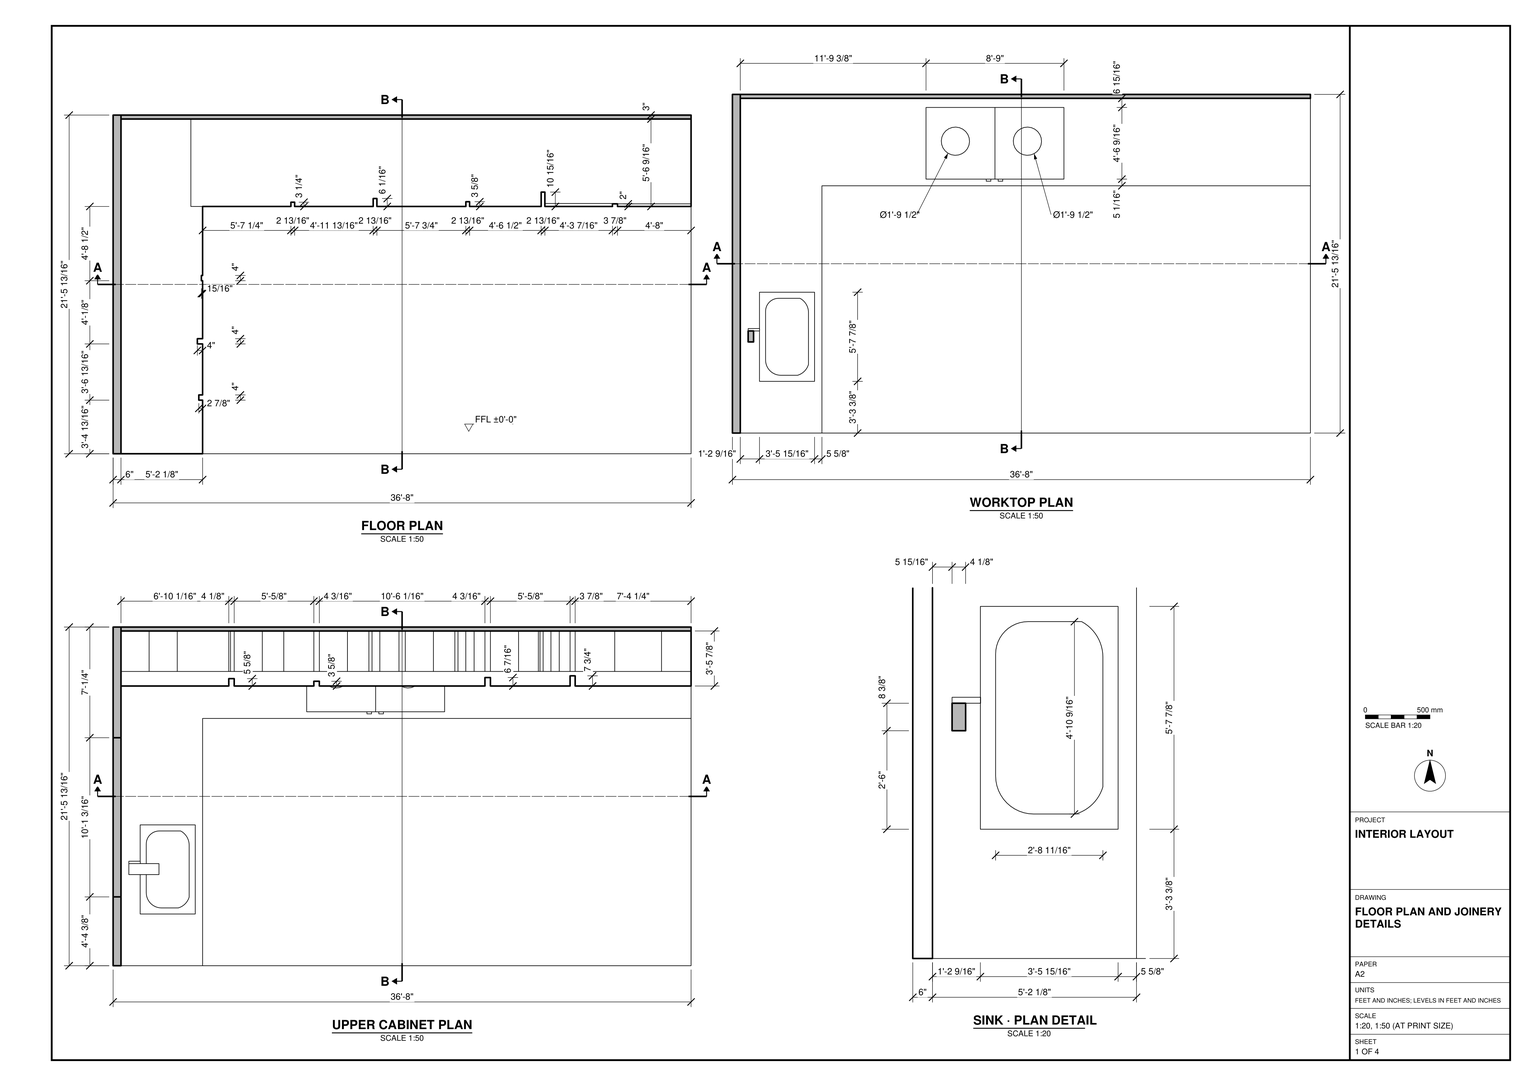
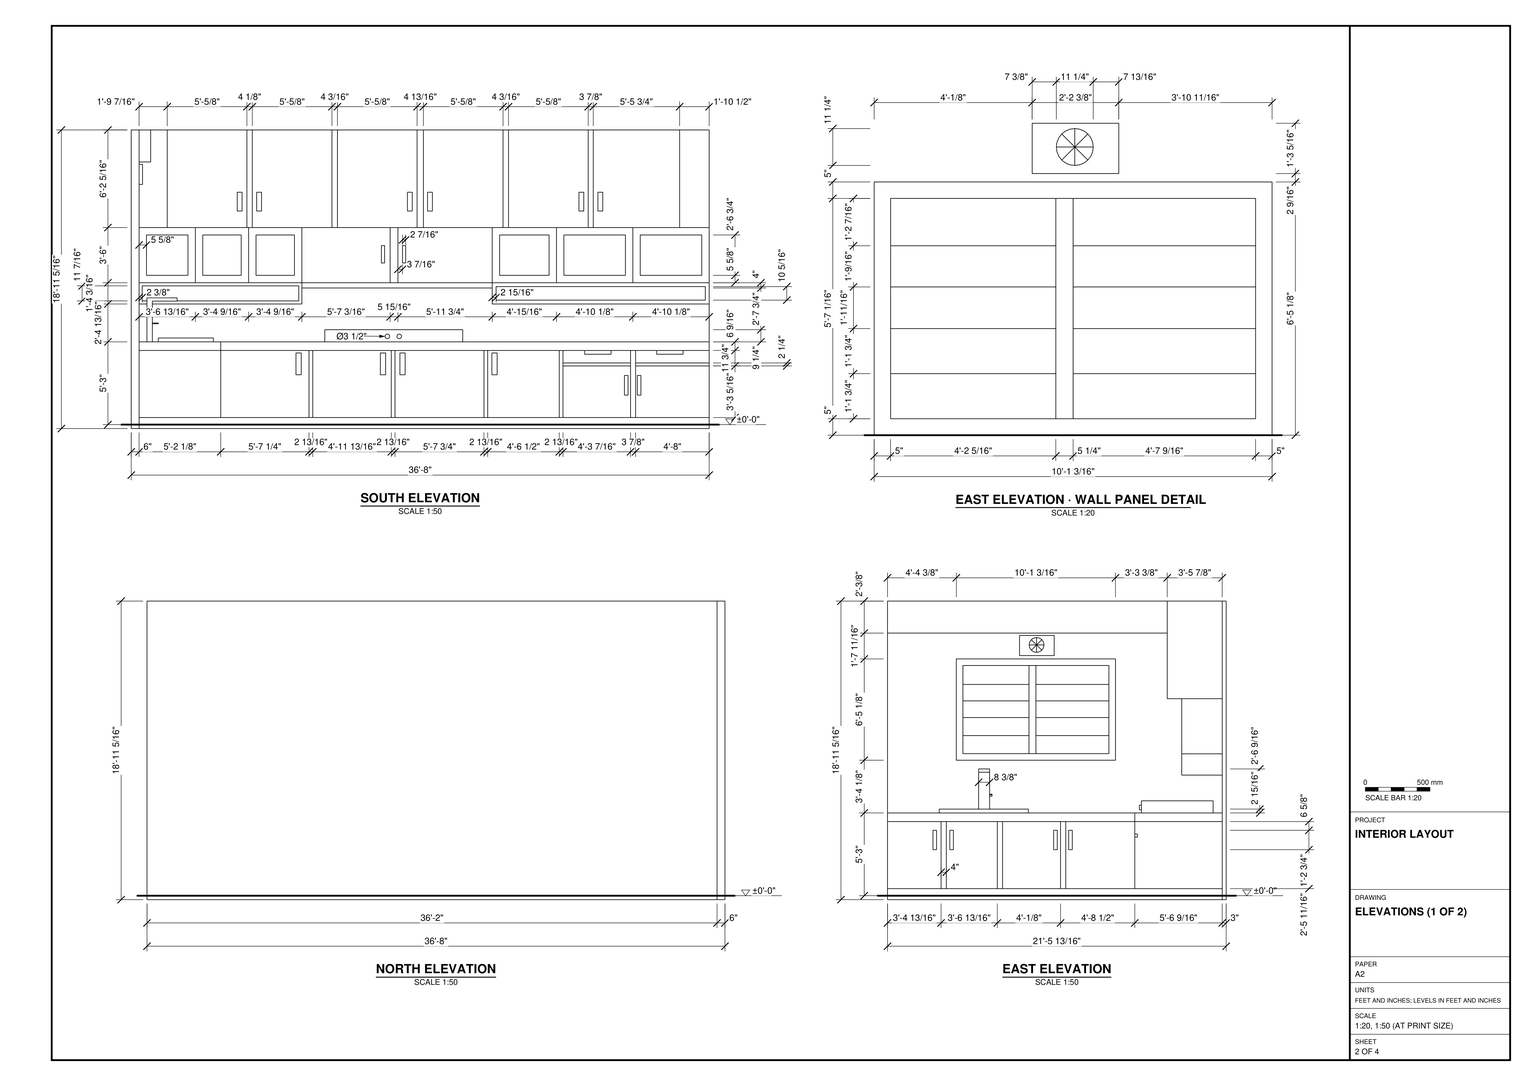
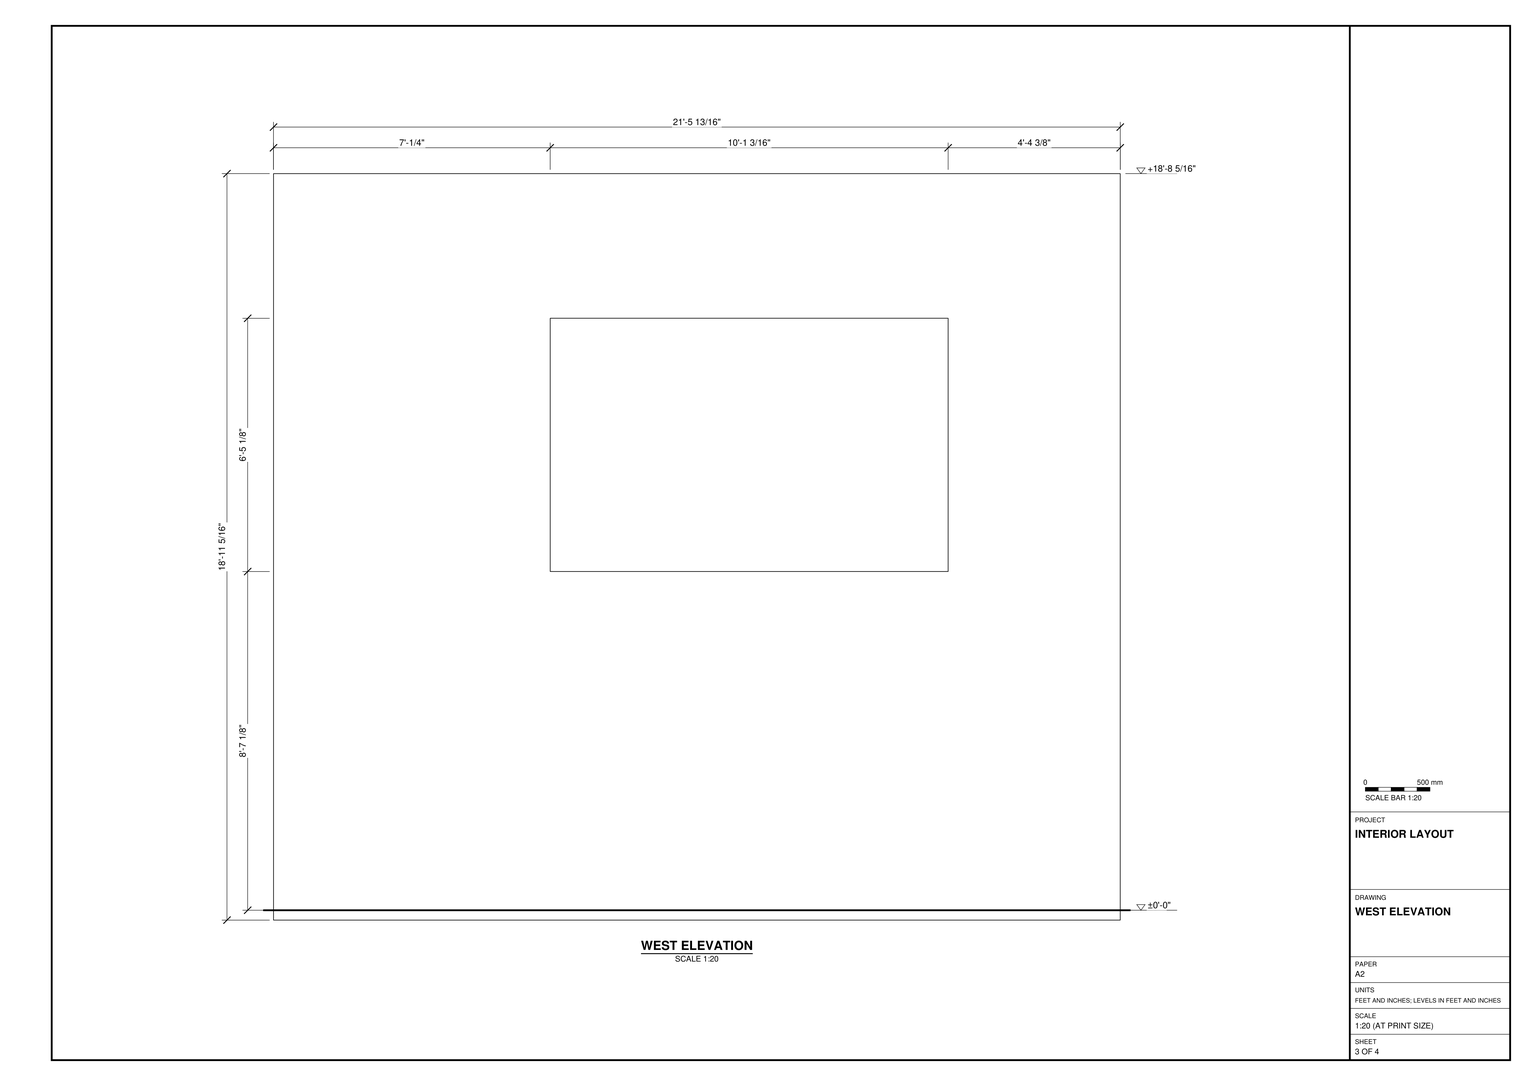
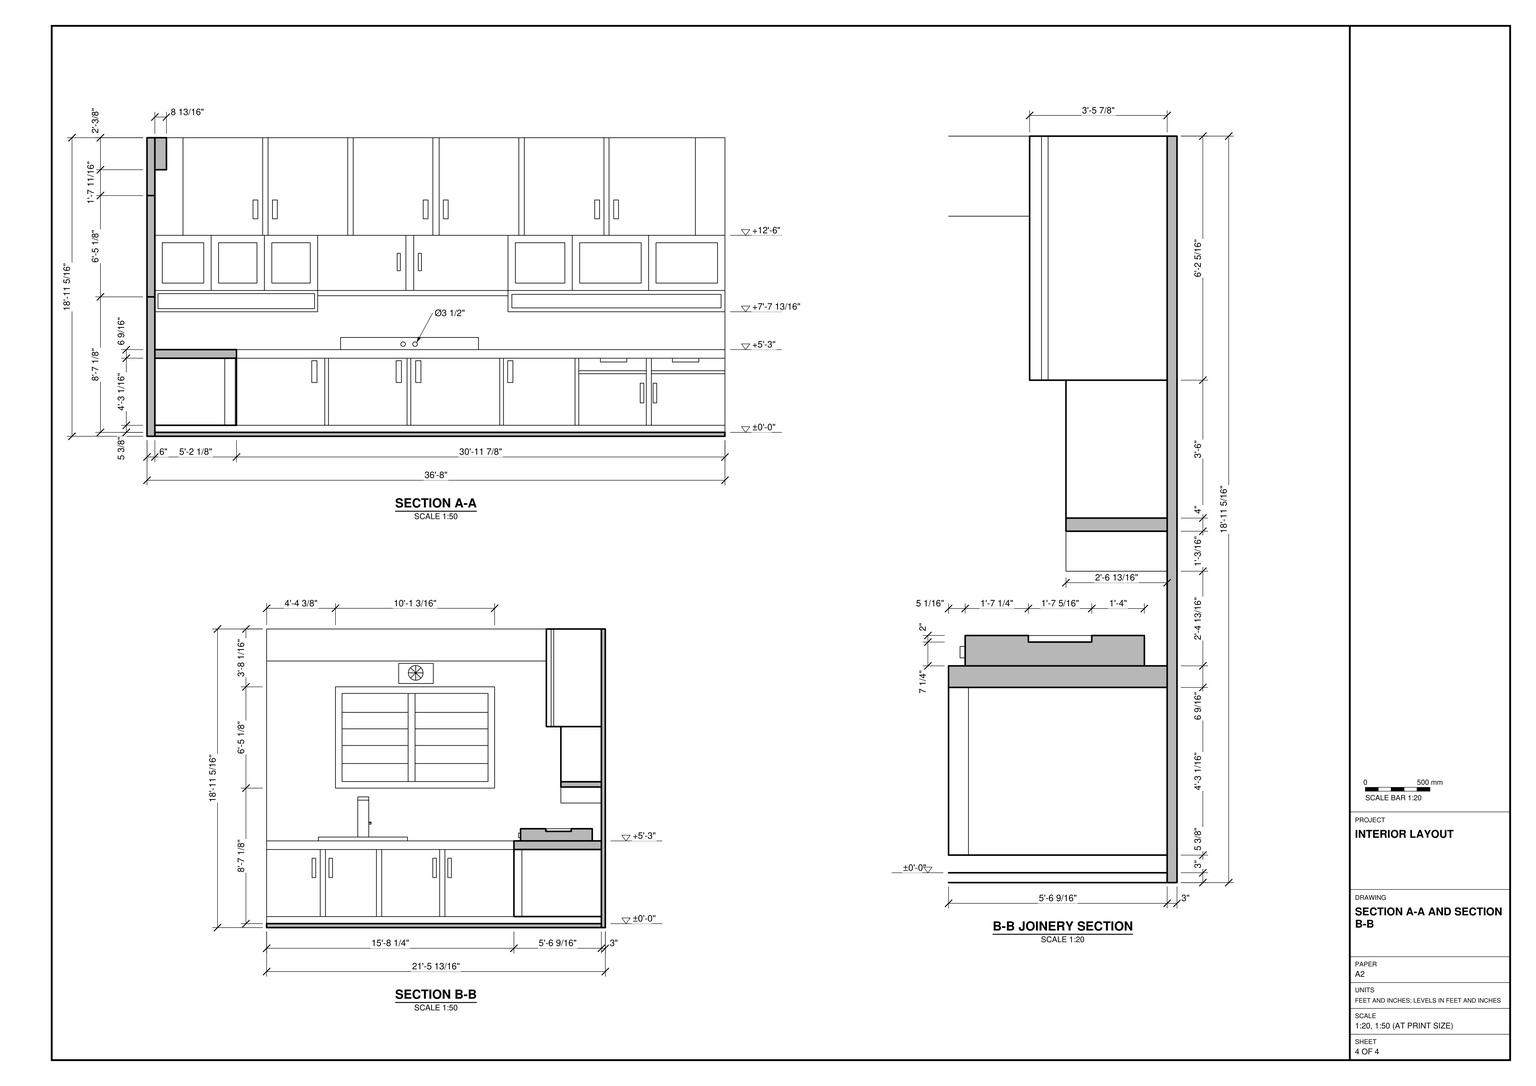
Build the kitchen interior in SketchUp from task_files/diagram_01.pdf. Work in feet and inches. Set the finished floor level to ±0'-0". The overall model extents are 36'-8" along the long cabinet wall, 21'-5 13/16" along the return and 18'-11 5/16" from bottom to top.

Model the rectangular floor slab and the two adjoining walls shown in plan. Make the long back wall 3" thick and the left return wall 6" thick. Follow the floor and worktop plans to form an L-shaped counter with base cabinets beneath both runs. Match the cabinet divisions, plinths, doors, drawer fronts and pulls to the elevations. Place the sink and tap on the return and the cooktop on the long run. Above the sink, model the framed wall panel with its central upright and horizontal divisions, and place the small wall fitting above it.

Use the upper cabinet plan for the depth and spacing of the wall units and the south elevation for their fronts. Distinguish the tall upper doors from the lower tier of framed and plain fronts and the open recesses beneath them. Keep the slab, walls and individual joinery pieces in separate groups or components, and use components for repeated parts. Decor, loose items and appliances may be any suitable library components. Save one SketchUp model as output_files/l_shaped_kitchen_interior_with_fitted_cabinetry.skp.

# SketchUp Ruby script. Lengths in inches.
U = 1.inch
M = Sketchup.active_model
def pt(a) = Geom::Point3d.new(a.map { |v| v * U })
def face(e, loops, mat)
  f = e.add_face(loops[0].map { |a| pt(a) })
  loops[1..].each { |l| e.add_face(l.map { |a| pt(a) }).erase! }
  f.material = f.back_material = mat if mat
  f
end
# faces: each face lists its corners as indices into pts; further lists are holes
def faces(e, pts, list, mat = nil) = list.each { |f| face(e, (f[0].is_a?(Array) ? f : [f]).map { |l| l.map { |i| pts[i] } }, mat) }
# xy, xz, yz: faces in a plane at the given z, y or x. An outline is a flat list of corners, or four numbers for a rectangle; further outlines are holes
def ring(l) = l.size == 4 ? [[l[0], l[1]], [l[2], l[1]], [l[2], l[3]], [l[0], l[3]]] : l.each_slice(2).to_a
def flat(e, list, mat, &to3) = list.each { |f| face(e, (f[0].is_a?(Array) ? f : [f]).map { |l| ring(l).map { |u, v| to3.(u, v) } }, mat) }
def xy(e, z, list, mat = nil) = flat(e, list, mat) { |x, y| [x, y, z] }
def xz(e, y, list, mat = nil) = flat(e, list, mat) { |x, z| [x, y, z] }
def yz(e, x, list, mat = nil) = flat(e, list, mat) { |y, z| [x, y, z] }
def lines(e, pts, list) = list.each { |a, b| e.add_line(pt(pts[a]), pt(pts[b])) }
# prism: a flat outline (further loops are holes) pulled along v
def prism(e, loops, v, mat = nil)
  f = face(e, loops, mat); d = Geom::Vector3d.new(v.map { |x| x * U })
  f.pushpull(f.normal.samedirection?(d) ? d.length : -d.length)
end
def box(e, o, s, mat = nil) = prism(e, [[o, [o[0] + s[0], o[1], o[2]], [o[0] + s[0], o[1] + s[1], o[2]], [o[0], o[1] + s[1], o[2]]]], [0, 0, s[2]], mat)
def at(x, y, z, deg = 0) = Geom::Transformation.translation(pt([x, y, z])) * Geom::Transformation.rotation(ORIGIN, Z_AXIS, deg.degrees)
def axes(o, x, y, z) = Geom::Transformation.new([*x, 0, *y, 0, *z, 0, *pt(o).to_a, 1])
def part(name) = M.definitions.add(name)
# library, detail: a bought-in or finely detailed component or shape, given as its bounding box
def library(name, o, s) = part(name).tap { |d| box(d.entities, o, s) }
def detail(e, o, s) = box(e.add_group.entities, o, s)
def put(e, d, t, mat = nil) = e.add_instance(d, t).tap { |i| i.material = mat if mat }
def group(e, t, mat = nil) = e.add_group.tap { |g| g.transformation = t; g.material = mat if mat }.entities
root = M.entities
M.materials.add("[Color M00]").color = [255, 255, 255]
M.materials.add("[Color M01]").color = [226, 226, 226]
M.materials.add("[Color M03]").color = [170, 170, 170]
M.materials.add("[Formica Graystone]").color = [149, 146, 135]
M.materials.add("[Formica Laminate Dark]").color = [50, 53, 60]
M.materials.add("[Formica Speckled Grey]").color = [94, 105, 111]
M.materials.add("[Quartz Light Brown]").color = [199, 184, 152]
M.materials.add("[Terrazzo Tile Light]").color = [219, 217, 210]
M.materials.add("[Tile Canvas]").color = [199, 192, 173]
M.materials.add("[Tile Ceramic Natural]").color = [189, 180, 134]
M.materials.add("[Tile Limestone Multi]").color = [199, 173, 118]
M.materials.add("[Translucent Glass Gray]").color = [128, 128, 128]
M.materials["[Translucent Glass Gray]"].alpha = 0.5
M.materials.add("[Translucent Glass Safety]").color = [204, 235, 244]
M.materials["[Translucent Glass Safety]"].alpha = 0.5
M.materials.add("[Wood Bamboo]").color = [177, 105, 43]
M.materials.add("[Wood Cherry Original]").color = [152, 86, 42]
M.materials.add("[Wood Floor Light]").color = [204, 176, 127]
xy(root,0,[[0,0,6,257.82],[6,0,439.97,254.82],[6,254.82,439.97,257.82]])
xy(root,3,[[6,0,439.97,254.82]],"[Tile Ceramic Natural]")
xy(root,8.375,[[6,0,6,254.82,59.1875,254.82,59.1875,188.26,68.125,188.26,68.125,135.72,67.1875,135.72,67.1875,131.74,68.125,131.74,68.125,87.6,64.125,87.6,64.125,83.61,68.125,83.61,68.125,44.78,65.25,44.78,65.25,40.8,68.125,40.8,68.125,0],[59.1875,188.26,59.1875,254.82,439.97,254.82,439.97,188.26,383.97,188.26,383.97,190.26,380.12,190.26,380.12,188.26,328.68,188.26,328.68,199.2,325.86,199.2,325.86,188.26,271.37,188.26,271.37,191.88,268.54,191.88,268.54,188.26,200.81,188.26,200.81,194.32,197.98,194.32,197.98,188.26,138.18,188.26,138.18,191.51,135.36,191.51,135.36,188.26]])
xy(root,47.66,[[328.68,188.26,380.12,190.51],[383.97,188.26,439.97,190.26]],"[Formica Laminate Dark]")
xy(root,49.93,[[328.68,188.26,380.12,190.51],[383.97,188.26,439.97,190.26]],"[Formica Laminate Dark]")
xy(root,50.5,[[36.81,44,49.6,44,50.5625,44.33,51.5,44.73,52.4,45.22,53.25,45.77,54.06,46.4,54.81,47.09,55.5,47.84,56.12,48.64,56.68,49.5,57.16,50.4,57.57,51.33,57.89,52.3,57.89,91.75,57.84,92.86,57.7,93.95,57.45,95.03,57.11,96.07,56.68,97.09,56.16,98.0625,55.55,98.98,54.86,99.85,54.1,100.65,53.27,101.37,52.38,102.02,51.4375,102.59,35.11,102.59,33.82,102.51,32.55,102.25,31.32,101.84,30.17,101.27,29.09,100.55,28.12,99.7,27.27,98.72,26.55,97.65,25.98,96.49,25.56,95.26,25.31,94,25.22,92.71,25.22,55.59,25.32,54.08,25.62,52.59,26.11,51.16,26.78,49.8,27.62,48.54,28.62,47.4,29.76,46.4,31.02,45.55,32.38,44.88,33.8125,44.4,35.3,44.1]])
xy(root,59.4375,[[6,0,6,254.82,439.97,254.82,439.97,188.26,383.97,188.26,383.97,190.26,380.12,190.26,380.12,188.26,328.68,188.26,328.68,199.2,325.86,199.2,325.86,188.26,271.37,188.26,271.37,191.88,268.54,191.88,268.54,188.26,200.81,188.26,200.81,194.32,197.98,194.32,197.98,188.26,138.18,188.26,138.18,191.51,135.36,191.51,135.36,188.26,68.125,188.26,68.125,135.72,67.1875,135.72,67.1875,131.74,68.125,131.74,68.125,87.6,64.125,87.6,64.125,83.61,68.125,83.61,68.125,44.78,65.25,44.78,65.25,40.8,68.125,40.8,68.125,0]],"[Color M03]")
xy(root,59.4375,[[65.25,40.8,68.125,44.78],[64.125,83.61,68.125,87.6],[67.1875,131.74,68.125,135.72],[135.36,188.26,138.18,191.51],[197.98,188.26,200.81,194.32],
  [268.54,188.26,271.37,191.88],[325.86,188.26,328.68,199.2],[380.12,188.26,383.97,190.26]],"[Formica Laminate Dark]")
xy(root,66,[[[20.59,39.37,62.53,107.22],[36.81,44,49.6,44,50.5625,44.33,51.5,44.73,52.4,45.22,53.25,45.77,54.06,46.4,54.81,47.09,55.5,47.84,56.12,48.64,56.68,49.5,57.16,50.4,57.57,51.33,57.89,52.3,57.89,91.75,57.84,92.86,57.7,93.95,57.45,95.03,57.11,96.07,56.68,97.09,56.16,98.0625,55.55,98.98,54.86,99.85,54.1,100.65,53.27,101.37,52.38,102.02,51.4375,102.59,35.11,102.59,33.82,102.51,32.55,102.25,31.32,101.84,30.17,101.27,29.09,100.55,28.12,99.7,27.27,98.72,26.55,97.65,25.98,96.49,25.56,95.26,25.31,94,25.22,92.71,25.22,55.59,25.32,54.08,25.62,52.59,26.11,51.16,26.78,49.8,27.62,48.54,28.62,47.4,29.76,46.4,31.02,45.55,32.38,44.88,33.8125,44.4,35.3,44.1]],[11.97,69.36,16.09,77.74],[147.37,193.32,252.37,247.88]])
xy(root,66,[[[6,0,68.125,0,68.125,188.26,439.97,188.26,439.97,254.82,6,254.82],[147.37,193.32,252.37,247.88],[20.59,39.37,62.53,107.22],[11.97,69.36,16.09,77.74]]],"[Formica Laminate Dark]")
xy(root,68.9375,[[[20.59,39.37,62.53,107.22],[36.81,44,35.3,44.1,33.8125,44.4,32.38,44.88,31.02,45.55,29.76,46.4,28.62,47.4,27.62,48.54,26.78,49.8,26.11,51.16,25.62,52.59,25.32,54.08,25.22,55.59,25.22,92.71,25.31,94,25.56,95.26,25.98,96.49,26.55,97.65,27.27,98.72,28.12,99.7,29.09,100.55,30.17,101.27,31.32,101.84,32.55,102.25,33.82,102.51,35.11,102.59,51.4375,102.59,52.38,102.02,53.27,101.37,54.1,100.65,54.86,99.85,55.55,98.98,56.16,98.0625,56.68,97.09,57.11,96.07,57.45,95.03,57.7,93.95,57.84,92.86,57.89,91.75,57.89,52.3,57.57,51.33,57.16,50.4,56.68,49.5,56.12,48.64,55.5,47.84,54.81,47.09,54.06,46.4,53.25,45.77,52.4,45.22,51.5,44.73,50.5625,44.33,49.6,44]]],"[Formica Graystone]")
xy(root,73.25,[[169.4375,211.46,172.23,211.74,174.85,212.74,177.125,214.39,178.9,216.5625,180.04,219.125,180.49,221.89,180.2,224.6875,179.2,227.31,177.56,229.58,175.38,231.35,172.82,232.5,170.05,232.95,167.26,232.66,164.64,231.66,162.36,230.02,160.59,227.84,159.44,225.28,159,222.51,159.28,219.72,160.28,217.09,161.93,214.82,164.11,213.05,166.67,211.9],[224.25,211.46,227.04,211.74,229.66,212.74,231.9375,214.39,233.71,216.5625,234.86,219.125,235.3,221.89,235.01,224.6875,234.01,227.31,232.37,229.58,230.19,231.35,227.63,232.5,224.86,232.95,222.07,232.66,219.45,231.66,217.17,230.02,215.4,227.84,214.26,225.28,213.81,222.51,214.1,219.72,215.1,217.09,216.74,214.82,218.92,213.05,221.48,211.9]],"[Formica Speckled Grey]")
xy(root,75.25,[[[147.37,193.32,199.87,247.88],[169.4375,211.46,166.67,211.9,164.11,213.05,161.93,214.82,160.28,217.09,159.28,219.72,159,222.51,159.44,225.28,160.59,227.84,162.36,230.02,164.64,231.66,167.26,232.66,170.05,232.95,172.82,232.5,175.38,231.35,177.56,229.58,179.2,227.31,180.2,224.6875,180.49,221.89,180.04,219.125,178.9,216.5625,177.125,214.39,174.85,212.74,172.23,211.74]],[[199.87,193.32,252.37,247.88],[224.25,211.46,221.48,211.9,218.92,213.05,216.74,214.82,215.1,217.09,214.1,219.72,213.81,222.51,214.26,225.28,215.4,227.84,217.17,230.02,219.45,231.66,222.07,232.66,224.86,232.95,227.63,232.5,230.19,231.35,232.37,229.58,234.01,227.31,235.01,224.6875,235.3,221.89,234.86,219.125,233.71,216.5625,231.9375,214.39,229.66,212.74,227.04,211.74]]],"[Formica Graystone]")
xy(root,78.75,[[11.97,77.74,16.09,79.55]])
xy(root,79.75,[[16.09,77.74,20.66,79.55]])
xy(root,80.32,[[11.97,77.74,20.66,79.55]],"[Terrazzo Tile Light]")
xy(root,94.8125,[[6,224.01,129.3125,254.82],[129.3125,224.01,129.91,254.82],[274.81,224.01,439.97,254.82]],"[Wood Cherry Original]")
xy(root,96.99,[[16.09,69.36,34.91,77.74]],"[Terrazzo Tile Light]")
xy(root,97.18,[[8.37,224.01,127.55,254.82]],"[Wood Cherry Original]")
xy(root,97.76,[[277.76,224.01,437.03,254.82]],"[Wood Cherry Original]")
xy(root,99.5,[[11.97,69.36,34.91,77.74]],"[Terrazzo Tile Light]")
xy(root,106.15,[[0,52.4,6,173.57]])
xy(root,107,[[129.91,224.01,274.81,254.82]],"[Color M00]")
xy(root,108.05,[[277.76,224.01,323.74,254.82],[323.74,224.01,381.86,254.82],[381.86,224.01,437.03,254.82]],"[Wood Cherry Original]")
xy(root,108.63,[[8.37,224.01,48.84,254.82],[48.84,224.01,89.375,254.82],[89.375,224.01,127.55,254.82]],"[Wood Cherry Original]")
xy(root,111,[[6,224.01,48.84,254.82],[48.84,224.01,89.375,254.82],[89.375,224.01,129.91,254.82],[129.91,224.01,274.81,254.82],[274.81,224.01,323.74,254.82],
  [323.74,224.01,381.86,254.82],[381.86,224.01,439.97,254.82]])
xy(root,116.64,[[11.64,224.01,43.2,254.82],[54.47,224.01,83.74,254.82],[95.01,224.01,124.28,254.82],[280.45,224.01,318.1,254.82],[329.37,224.01,376.22,254.82],
  [387.49,224.01,434.34,254.82]],"[Wood Bamboo]")
xy(root,147.36,[[11.64,224.01,43.2,254.82],[54.47,224.01,83.74,254.82],[95.01,224.01,124.28,254.82],[280.45,224.01,318.1,254.82],[329.37,224.01,376.22,254.82],
  [387.49,224.01,434.34,254.82]],"[Wood Bamboo]")
xy(root,153,[[6,224.01,27.42,254.82],[27.42,224.01,48.84,254.82],[48.84,224.01,88.0625,254.82],[88.0625,224.01,89.375,254.82],[89.375,224.01,92.17,254.82],
  [92.17,224.01,113.59,254.82],[113.59,224.01,129.91,254.82],[129.91,224.01,152.8125,254.82],[152.8125,224.01,156.98,254.82],[156.98,224.01,178.4,254.82],
  [178.4,224.01,194.73,254.82],[194.73,224.01,197.1,254.82],[197.1,224.01,203.05,254.82],[203.05,224.01,217.625,254.82],[217.625,224.01,222.42,254.82],
  [222.42,224.01,243.84,254.82],[243.84,224.01,260.16,254.82],[260.16,224.01,262.54,254.82],[262.54,224.01,268.49,254.82],[268.49,224.01,274.81,254.82],
  [274.81,224.01,283.0625,254.82],[283.0625,224.01,287.23,254.82],[287.23,224.01,308.65,254.82],[308.65,224.01,323.74,254.82],[323.74,224.01,324.98,254.82],
  [324.98,224.01,327.35,254.82],[327.35,224.01,333.3,254.82],[333.3,224.01,339.63,254.82],[339.63,224.01,347.875,254.82],[347.875,224.01,351.74,254.82],
  [351.74,224.01,381.86,254.82],[381.86,224.01,417.48,254.82],[417.48,224.01,439.97,254.82]])
xy(root,153,[[6,212.95,6,224.01,439.97,224.01,439.97,212.95,351.74,212.95,351.74,220.7,347.875,220.7,347.875,212.95,287.23,212.95,287.23,219.38,283.0625,219.38,283.0625,212.95,156.98,212.95,156.98,216.57,152.8125,216.57,152.8125,212.95,92.17,212.95,92.17,218.57,88.0625,218.57,88.0625,212.95]],"[Wood Bamboo]")
xy(root,183.28,[[0,52.4,6,173.57]])
xy(root,185.83,[[6,100.52,8.625,126.9]],"[Color M01]")
xy(root,201.14,[[6,100.52,8.625,126.9]],"[Color M01]")
xy(root,202.9375,[[6,0,14.8125,212.95]])
xy(root,227.3125,[[6,254.82,439.97,257.82]])
xy(root,227.3125,[[6,0,14.8125,212.95]],"[Color M00]")
xy(root,227.3125,[[0,0,6,257.82]],"[Tile Canvas]")
xy(root,227.3125,[[6,212.95,27.42,254.82],[27.42,212.95,88.0625,254.82],[92.17,212.95,152.8125,254.82],[156.98,212.95,217.625,254.82],[217.625,212.95,222.42,254.82],
  [222.42,212.95,283.0625,254.82],[287.23,212.95,347.875,254.82],[351.74,212.95,417.48,254.82],[417.48,212.95,439.97,254.82],[152.8125,216.57,156.98,254.82],
  [88.0625,218.57,92.17,254.82],[283.0625,219.38,287.23,254.82],[347.875,220.7,351.74,254.82]],"[Wood Bamboo]")
xz(root,0,[[6,202.9375,14.8125,227.3125]],"[Color M00]")
xz(root,0,[[6,59.4375,68.125,66]],"[Formica Laminate Dark]")
xz(root,0,[[0,0,6,227.3125],[6,0,439.97,3]],"[Tile Canvas]")
xz(root,0,[[6,8.375,68.125,59.4375]],"[Wood Cherry Original]")
xz(root,39.37,[[20.59,66,62.53,68.9375]],"[Formica Graystone]")
xz(root,40.8,[[65.25,8.375,68.125,59.4375]],"[Formica Laminate Dark]")
xz(root,44,[[36.81,50.5,49.6,66],[36.81,66,49.6,68.9375]],"[Formica Graystone]")
xz(root,44.78,[[65.25,8.375,68.125,59.4375]],"[Formica Laminate Dark]")
xz(root,52.4,[[0,106.15,6,183.28]])
xz(root,69.36,[[11.97,66,16.09,66,16.09,96.99,34.91,96.99,34.91,99.5,11.97,99.5]],"[Terrazzo Tile Light]")
xz(root,77.74,[[11.97,78.75,16.09,80.32]])
xz(root,77.74,[[11.97,66,16.09,78.75],[16.09,79.75,20.66,80.32],[11.97,80.32,11.97,99.5,34.91,99.5,34.91,96.99,16.09,96.99,16.09,80.32]],"[Terrazzo Tile Light]")
xz(root,79.55,[[11.97,78.75,11.97,80.32,20.66,80.32,20.66,79.75,16.09,79.75,16.09,78.75]],"[Terrazzo Tile Light]")
xz(root,83.61,[[64.125,8.375,68.125,59.4375]],"[Formica Laminate Dark]")
xz(root,87.6,[[64.125,8.375,68.125,59.4375]],"[Formica Laminate Dark]")
xz(root,100.52,[[6,185.83,8.625,201.14]],"[Color M01]")
xz(root,102.59,[[35.11,50.5,51.4375,66],[35.11,66,51.4375,68.9375]],"[Formica Graystone]")
xz(root,107.22,[[20.59,66,62.53,68.9375]],"[Formica Graystone]")
xz(root,126.9,[[6,185.83,8.625,201.14]],"[Color M01]")
xz(root,131.74,[[67.1875,8.375,68.125,59.4375]],"[Formica Laminate Dark]")
xz(root,135.72,[[67.1875,8.375,68.125,59.4375]],"[Formica Laminate Dark]")
xz(root,173.57,[[0,106.15,6,183.28]])
xz(root,188.26,[[68.125,59.4375,439.97,66]],"[Formica Laminate Dark]")
xz(root,188.26,[[[68.125,8.375,135.36,59.4375],[125.43,40.93,129.43,57.55]],[[138.18,8.375,197.98,59.4375],[189.68,40.93,193.68,57.55]],[[200.81,8.375,268.54,59.4375],[204.55,40.93,208.55,57.55]],[[271.37,8.375,325.86,59.4375],[274.55,40.93,278.55,57.55]],[[328.68,8.375,380.12,47.66],[375.47,25.42,378.22,40.42]],
  [[383.97,8.375,439.97,47.66],[385.28,25.42,388.03,40.42]],[328.68,49.93,380.12,49.93,380.12,59.4375,365.3,59.4375,365.3,56.5625,345.17,56.5625,345.17,59.4375,328.68,59.4375],[383.97,49.93,439.97,49.93,439.97,59.4375,420.11,59.4375,420.11,56.5625,399.99,56.5625,399.99,59.4375,383.97,59.4375]],"[Wood Cherry Original]")
xz(root,188.26,[[375.47,25.42,378.22,40.42],[385.28,25.42,388.03,40.42],[125.43,40.93,129.43,57.55],[189.68,40.93,193.68,57.55],[204.55,40.93,208.55,57.55],
  [274.55,40.93,278.55,57.55],[345.17,56.5625,365.3,59.4375],[399.99,56.5625,420.11,59.4375]],"[Wood Floor Light]")
xz(root,190.26,[[380.12,8.375,383.97,59.4375],[383.97,47.66,439.97,49.93]],"[Formica Laminate Dark]")
xz(root,190.51,[[328.68,47.66,380.12,49.93]],"[Formica Laminate Dark]")
xz(root,191.51,[[135.36,8.375,138.18,59.4375]],"[Formica Laminate Dark]")
xz(root,191.75,[[194.97,68.43,195.42,68.49,195.84,68.66,196.21,68.94,196.49,69.3,196.66,69.72,196.72,70.18,196.66,70.63,196.49,71.05,196.21,71.42,195.84,71.69,195.42,71.87,194.97,71.93,194.52,71.87,194.09,71.69,193.73,71.42,193.45,71.05,193.28,70.63,193.22,70.18,193.28,69.72,193.45,69.3,193.73,68.94,194.09,68.66,194.52,68.49],[204.03,68.43,204.49,68.49,204.91,68.66,205.27,68.94,205.55,69.3,205.72,69.72,205.78,70.18,205.72,70.63,205.55,71.05,205.27,71.42,204.91,71.69,204.49,71.87,204.03,71.93,203.58,71.87,203.16,71.69,202.79,71.42,202.52,71.05,202.34,70.63,202.28,70.18,202.34,69.72,202.52,69.3,202.79,68.94,203.16,68.66,203.58,68.49]],"[Formica Laminate Dark]")
xz(root,191.88,[[268.54,8.375,271.37,59.4375]],"[Formica Laminate Dark]")
xz(root,193.32,[[194.97,68.43,194.52,68.49,194.09,68.66,193.73,68.94,193.45,69.3,193.28,69.72,193.22,70.18,193.28,70.63,193.45,71.05,193.73,71.42,194.09,71.69,194.52,71.87,194.97,71.93,195.42,71.87,195.84,71.69,196.21,71.42,196.49,71.05,196.66,70.63,196.72,70.18,196.66,69.72,196.49,69.3,196.21,68.94,195.84,68.66,195.42,68.49],[204.03,68.43,203.58,68.49,203.16,68.66,202.79,68.94,202.52,69.3,202.34,69.72,202.28,70.18,202.34,70.63,202.52,71.05,202.79,71.42,203.16,71.69,203.58,71.87,204.03,71.93,204.49,71.87,204.91,71.69,205.27,71.42,205.55,71.05,205.72,70.63,205.78,70.18,205.72,69.72,205.55,69.3,205.27,68.94,204.91,68.66,204.49,68.49]])
xz(root,193.32,[[[147.37,66,252.37,75.25],[194.97,68.43,194.52,68.49,194.09,68.66,193.73,68.94,193.45,69.3,193.28,69.72,193.22,70.18,193.28,70.63,193.45,71.05,193.73,71.42,194.09,71.69,194.52,71.87,194.97,71.93,195.42,71.87,195.84,71.69,196.21,71.42,196.49,71.05,196.66,70.63,196.72,70.18,196.66,69.72,196.49,69.3,196.21,68.94,195.84,68.66,195.42,68.49],[204.03,68.43,203.58,68.49,203.16,68.66,202.79,68.94,202.52,69.3,202.34,69.72,202.28,70.18,202.34,70.63,202.52,71.05,202.79,71.42,203.16,71.69,203.58,71.87,204.03,71.93,204.49,71.87,204.91,71.69,205.27,71.42,205.55,71.05,205.72,70.63,205.78,70.18,205.72,69.72,205.55,69.3,205.27,68.94,204.91,68.66,204.49,68.49]]],"[Formica Graystone]")
xz(root,194.32,[[197.98,8.375,200.81,59.4375]],"[Formica Laminate Dark]")
xz(root,199.2,[[325.86,8.375,328.68,59.4375]],"[Formica Laminate Dark]")
xz(root,212.95,[[6,202.9375,14.8125,227.3125]])
xz(root,212.95,[[217.625,153,222.42,227.3125]],"[Formica Laminate Dark]")
xz(root,212.95,[[6,153,27.42,153,27.42,227.3125,14.8125,227.3125,14.8125,202.9375,6,202.9375],[[27.42,153,88.0625,227.3125],[80.71,165.59,84.4,179.9]],[[92.17,153,152.8125,227.3125],[95.52,165.59,99.21,179.9]],[[156.98,153,217.625,227.3125],[210.27,165.59,213.96,179.9]],[[222.42,153,283.0625,227.3125],[225.58,165.59,229.27,179.9]],
  [[287.23,153,347.875,227.3125],[340.83,165.59,344.52,179.9]],[[351.74,153,417.48,227.3125],[355.27,165.59,358.96,179.9]],[417.48,153,439.97,227.3125]],"[Wood Bamboo]")
xz(root,212.95,[[80.71,165.59,84.4,179.9],[95.52,165.59,99.21,179.9],[210.27,165.59,213.96,179.9],[225.58,165.59,229.27,179.9],[340.83,165.59,344.52,179.9],
  [355.27,165.59,358.96,179.9]],"[Wood Floor Light]")
xz(root,216.57,[[152.8125,153,156.98,227.3125]],"[Formica Laminate Dark]")
xz(root,218.57,[[88.0625,153,92.17,227.3125]],"[Formica Laminate Dark]")
xz(root,219.38,[[283.0625,153,287.23,227.3125]],"[Formica Laminate Dark]")
xz(root,220.7,[[347.875,153,351.74,227.3125]],"[Formica Laminate Dark]")
xz(root,224.01,[[129.91,107,274.81,111]],"[Color M00]")
xz(root,224.01,[[197.1,111,203.05,153]],"[Formica Laminate Dark]")
xz(root,224.01,[[11.64,116.64,43.2,147.36],[54.47,116.64,83.74,147.36],[95.01,116.64,124.28,147.36],[280.45,116.64,318.1,147.36],[329.37,116.64,376.22,147.36],
  [387.49,116.64,434.34,147.36]],"[Translucent Glass Safety]")
xz(root,224.01,[[[6,111,48.84,153],[11.64,116.64,43.2,147.36]],[[48.84,111,89.375,153],[54.47,116.64,83.74,147.36]],[[89.375,111,129.91,153],[95.01,116.64,124.28,147.36]],[[274.81,111,323.74,153],[280.45,116.64,318.1,147.36]],[[323.74,111,381.86,153],[329.37,116.64,376.22,147.36]],
  [[381.86,111,439.97,153],[387.49,116.64,434.34,147.36]]],"[Wood Bamboo]")
xz(root,224.01,[[[6,94.8125,129.91,111],[8.37,97.18,127.55,108.63]],[[274.81,94.8125,439.97,111],[277.76,97.76,437.03,108.05]],[[129.91,111,197.1,153],[190.46,126.04,192.89,139.29]],[[203.05,111,274.81,153],[206.52,126.04,208.96,139.29]]],"[Wood Cherry Original]")
xz(root,224.01,[[190.46,126.04,192.89,139.29],[206.52,126.04,208.96,139.29]],"[Wood Floor Light]")
xz(root,247.88,[[147.37,66,252.37,75.25]])
xz(root,254.82,[[6,0,439.97,3],[6,8.375,59.1875,59.4375],[59.1875,8.375,439.97,59.4375],[6,59.4375,59.1875,66],[59.1875,59.4375,439.97,66],
  [[6,94.8125,129.91,111],[8.37,97.18,127.55,108.63]],[[274.81,94.8125,439.97,111],[277.76,97.76,437.03,108.05]],[129.91,107,197.1,111],[197.1,107,203.05,111],[203.05,107,274.81,111],
  [[6,111,48.84,153],[11.64,116.64,43.2,147.36]],[[48.84,111,89.375,153],[54.47,116.64,83.74,147.36]],[[89.375,111,129.91,153],[95.01,116.64,124.28,147.36]],[129.91,111,197.1,153],[197.1,111,203.05,153],
  [203.05,111,274.81,153],[[274.81,111,323.74,153],[280.45,116.64,318.1,147.36]],[[323.74,111,381.86,153],[329.37,116.64,376.22,147.36]],[[381.86,111,439.97,153],[387.49,116.64,434.34,147.36]],[6,153,27.42,227.3125],
  [27.42,153,88.0625,227.3125],[88.0625,153,92.17,227.3125],[92.17,153,152.8125,227.3125],[152.8125,153,156.98,227.3125],[156.98,153,217.625,227.3125],
  [217.625,153,222.42,227.3125],[222.42,153,283.0625,227.3125],[283.0625,153,287.23,227.3125],[287.23,153,347.875,227.3125],[347.875,153,351.74,227.3125],
  [351.74,153,417.48,227.3125],[417.48,153,439.97,227.3125]])
xz(root,254.82,[[6,3,439.97,8.375],[6,66,439.97,66,439.97,94.8125,274.81,94.8125,274.81,107,129.91,107,129.91,94.8125,6,94.8125]],"[Tile Canvas]")
xz(root,254.82,[[11.64,116.64,43.2,147.36],[54.47,116.64,83.74,147.36],[95.01,116.64,124.28,147.36],[280.45,116.64,318.1,147.36],[329.37,116.64,376.22,147.36],
  [387.49,116.64,434.34,147.36]],"[Wood Bamboo]")
xz(root,254.82,[[8.37,97.18,127.55,108.63],[277.76,97.76,437.03,108.05]],"[Wood Cherry Original]")
xz(root,257.82,[[0,0,6,227.3125],[6,0,439.97,227.3125]],"[Tile Limestone Multi]")
yz(root,0,[[[0,0,257.82,227.3125],[52.4,106.15,173.57,183.28]],[52.4,106.15,173.57,183.28]],"[Tile Limestone Multi]")
yz(root,6,[[0,0,254.82,3],[254.82,0,257.82,227.3125],[0,8.375,254.82,59.4375],[0,59.4375,254.82,66],[224.01,94.8125,254.82,111],
  [224.01,111,254.82,153],[212.95,153,254.82,227.3125],[0,202.9375,212.95,227.3125]])
yz(root,6,[[100.52,185.83,126.9,201.14]],"[Color M01]")
yz(root,6,[[[52.4,106.15,173.57,183.28],[57.42,111.17,168.55,178.26]],[107.72,111.17,112.98,178.26]],"[Quartz Light Brown]")
yz(root,6,[[0,3,254.82,8.375],[[0,66,254.82,66,254.82,94.8125,224.01,94.8125,224.01,153,212.95,153,212.95,202.9375,0,202.9375],[52.4,106.15,173.57,183.28],[100.52,185.83,126.9,201.14]]],"[Tile Canvas]")
yz(root,6,[[57.42,111.17,107.72,124.9],[112.98,111.17,168.55,124.9],[57.42,124.9,107.72,138.625],[112.98,124.9,168.55,138.625],[57.42,138.625,107.72,151.31],
  [112.98,138.625,168.55,151.31],[57.42,151.31,107.72,163.84],[112.98,151.31,168.55,163.84],[57.42,163.84,107.72,178.26],[112.98,163.84,168.55,178.26]],"[Translucent Glass Gray]")
yz(root,8.37,[[224.01,97.18,254.82,108.63]],"[Wood Cherry Original]")
yz(root,8.625,[[[100.52,185.83,126.9,201.14],[113.49,188.29,112.04,188.49,110.68,189.05,109.51,189.94,108.62,191.11,108.06,192.46,107.87,193.92,108.06,195.375,108.62,196.73,109.51,197.9,110.68,198.79,112.04,199.35,113.49,199.54,114.95,199.35,116.3,198.79,117.47,197.9,118.36,196.73,118.92,195.375,119.12,193.92,118.92,192.46,118.36,191.11,117.47,189.94,116.3,189.05,114.95,188.49]],[113.49,188.29,113.49,193.92,109.51,189.94,110.68,189.05,112.04,188.49],[113.49,188.29,114.95,188.49,116.3,189.05,117.47,189.94,113.49,193.92],[109.51,189.94,113.49,193.92,107.87,193.92,108.06,192.46,108.62,191.11],[117.47,189.94,118.36,191.11,118.92,192.46,119.12,193.92,113.49,193.92],
  [107.87,193.92,113.49,193.92,109.51,197.9,108.62,196.73,108.06,195.375],[113.49,193.92,113.49,199.54,112.04,199.35,110.68,198.79,109.51,197.9],[113.49,193.92,117.47,197.9,116.3,198.79,114.95,199.35,113.49,199.54],[113.49,193.92,119.12,193.92,118.92,195.375,118.36,196.73,117.47,197.9]],"[Color M01]")
yz(root,11.64,[[224.01,116.64,254.82,147.36]],"[Wood Bamboo]")
yz(root,11.97,[[69.36,66,77.74,99.5],[77.74,78.75,79.55,80.32]],"[Terrazzo Tile Light]")
yz(root,14.8125,[[0,202.9375,212.95,227.3125]],"[Color M00]")
yz(root,16.09,[[69.36,66,77.74,96.99],[77.74,78.75,79.55,79.75]],"[Terrazzo Tile Light]")
yz(root,20.59,[[39.37,66,107.22,68.9375]],"[Formica Graystone]")
yz(root,20.66,[[77.74,79.75,79.55,80.32]])
yz(root,25.22,[[55.59,50.5,92.71,66],[55.59,66,92.71,68.9375]],"[Formica Graystone]")
yz(root,34.91,[[69.36,96.99,77.74,99.5]],"[Terrazzo Tile Light]")
yz(root,43.2,[[224.01,116.64,254.82,147.36]],"[Wood Bamboo]")
yz(root,48.84,[[224.01,111,254.82,153]])
yz(root,54.47,[[224.01,116.64,254.82,147.36]],"[Wood Bamboo]")
yz(root,57.89,[[52.3,50.5,91.75,66],[52.3,66,91.75,68.9375]],"[Formica Graystone]")
yz(root,62.53,[[39.37,66,107.22,68.9375]],"[Formica Graystone]")
yz(root,64.125,[[83.61,8.375,87.6,59.4375]],"[Formica Laminate Dark]")
yz(root,65.25,[[40.8,8.375,44.78,59.4375]],"[Formica Laminate Dark]")
yz(root,67.1875,[[131.74,8.375,135.72,59.4375]],"[Formica Laminate Dark]")
yz(root,68.125,[[0,59.4375,188.26,66]],"[Formica Laminate Dark]")
yz(root,68.125,[[[0,8.375,40.8,59.4375],[34.61,38.05,37.36,52.8]],[[44.78,8.375,83.61,59.4375],[47.43,38.05,50.18,52.8]],[[87.6,8.375,131.74,59.4375],[126.49,38.05,129.24,52.8]],[[135.72,8.375,188.26,59.4375],[137.93,38.05,140.68,52.8]]],"[Wood Cherry Original]")
yz(root,68.125,[[34.61,38.05,37.36,52.8],[47.43,38.05,50.18,52.8],[126.49,38.05,129.24,52.8],[137.93,38.05,140.68,52.8]],"[Wood Floor Light]")
yz(root,83.74,[[224.01,116.64,254.82,147.36]],"[Wood Bamboo]")
yz(root,88.0625,[[212.95,153,218.57,227.3125]],"[Formica Laminate Dark]")
yz(root,89.375,[[224.01,111,254.82,153]])
yz(root,92.17,[[212.95,153,218.57,227.3125]],"[Formica Laminate Dark]")
yz(root,95.01,[[224.01,116.64,254.82,147.36]],"[Wood Bamboo]")
yz(root,124.28,[[224.01,116.64,254.82,147.36]],"[Wood Bamboo]")
yz(root,127.55,[[224.01,97.18,254.82,108.63]],"[Wood Cherry Original]")
yz(root,129.91,[[224.01,107,254.82,111],[224.01,111,254.82,153]])
yz(root,129.91,[[224.01,94.8125,254.82,107]],"[Wood Cherry Original]")
yz(root,135.36,[[188.26,8.375,191.51,59.4375]],"[Formica Laminate Dark]")
yz(root,138.18,[[188.26,8.375,191.51,59.4375]],"[Formica Laminate Dark]")
yz(root,147.37,[[193.32,66,247.88,75.25]],"[Formica Graystone]")
yz(root,152.8125,[[212.95,153,216.57,227.3125]],"[Formica Laminate Dark]")
yz(root,156.98,[[212.95,153,216.57,227.3125]],"[Formica Laminate Dark]")
yz(root,197.98,[[188.26,8.375,194.32,59.4375]],"[Formica Laminate Dark]")
yz(root,200.81,[[188.26,8.375,194.32,59.4375]],"[Formica Laminate Dark]")
yz(root,252.37,[[193.32,66,247.88,75.25]],"[Formica Graystone]")
yz(root,268.54,[[188.26,8.375,191.88,59.4375]],"[Formica Laminate Dark]")
yz(root,271.37,[[188.26,8.375,191.88,59.4375]],"[Formica Laminate Dark]")
yz(root,274.81,[[224.01,107,254.82,111],[224.01,111,254.82,153]])
yz(root,274.81,[[224.01,94.8125,254.82,107]],"[Wood Cherry Original]")
yz(root,277.76,[[224.01,97.76,254.82,108.05]],"[Wood Cherry Original]")
yz(root,280.45,[[224.01,116.64,254.82,147.36]],"[Wood Bamboo]")
yz(root,283.0625,[[212.95,153,219.38,227.3125]],"[Formica Laminate Dark]")
yz(root,287.23,[[212.95,153,219.38,227.3125]],"[Formica Laminate Dark]")
yz(root,318.1,[[224.01,116.64,254.82,147.36]],"[Wood Bamboo]")
yz(root,323.74,[[224.01,111,254.82,153]])
yz(root,325.86,[[188.26,8.375,199.2,59.4375]],"[Formica Laminate Dark]")
yz(root,328.68,[[188.26,8.375,199.2,47.66],[190.51,47.66,199.2,49.93],[188.26,49.93,199.2,59.4375]],"[Formica Laminate Dark]")
yz(root,329.37,[[224.01,116.64,254.82,147.36]],"[Wood Bamboo]")
yz(root,347.875,[[212.95,153,220.7,227.3125]],"[Formica Laminate Dark]")
yz(root,351.74,[[212.95,153,220.7,227.3125]],"[Formica Laminate Dark]")
yz(root,376.22,[[224.01,116.64,254.82,147.36]],"[Wood Bamboo]")
yz(root,380.12,[[188.26,8.375,190.26,47.66],[190.26,47.66,190.51,49.93],[188.26,49.93,190.26,59.4375]],"[Formica Laminate Dark]")
yz(root,381.86,[[224.01,111,254.82,153]])
yz(root,383.97,[[188.26,8.375,190.26,47.66],[188.26,49.93,190.26,59.4375]],"[Formica Laminate Dark]")
yz(root,387.49,[[224.01,116.64,254.82,147.36]],"[Wood Bamboo]")
yz(root,434.34,[[224.01,116.64,254.82,147.36]],"[Wood Bamboo]")
yz(root,437.03,[[224.01,97.76,254.82,108.05]],"[Wood Cherry Original]")
yz(root,439.97,[[188.26,59.4375,254.82,66]],"[Formica Laminate Dark]")
yz(root,439.97,[[0,0,254.82,3],[254.82,0,257.82,227.3125]],"[Tile Canvas]")
yz(root,439.97,[[224.01,111,254.82,153],[212.95,153,254.82,227.3125]],"[Wood Bamboo]")
yz(root,439.97,[[188.26,8.375,254.82,8.375,254.82,59.4375,188.26,59.4375,188.26,49.93,190.26,49.93,190.26,47.66,188.26,47.66],[224.01,94.8125,254.82,111]],"[Wood Cherry Original]")
p = [[35.3,44.1,66],[36.81,44,66],[36.81,44,50.5],[35.3,44.1,50.5],[49.6,44,66],[50.5625,44.33,66],
  [50.5625,44.33,50.5],[49.6,44,50.5],[33.8125,44.4,66],[33.8125,44.4,50.5],[51.5,44.73,66],[51.5,44.73,50.5],
  [32.38,44.88,66],[32.38,44.88,50.5],[52.4,45.22,66],[52.4,45.22,50.5],[31.02,45.55,66],[31.02,45.55,50.5],
  [53.25,45.77,66],[53.25,45.77,50.5],[29.76,46.4,66],[29.76,46.4,50.5],[54.06,46.4,66],[54.06,46.4,50.5],
  [28.62,47.4,66],[28.62,47.4,50.5],[54.81,47.09,66],[54.81,47.09,50.5],[55.5,47.84,66],[55.5,47.84,50.5],
  [27.62,48.54,66],[27.62,48.54,50.5],[56.12,48.64,66],[56.12,48.64,50.5],[26.78,49.8,66],[26.78,49.8,50.5],
  [56.68,49.5,66],[56.68,49.5,50.5],[57.16,50.4,66],[57.16,50.4,50.5],[26.11,51.16,66],[26.11,51.16,50.5],
  [57.57,51.33,66],[57.57,51.33,50.5],[25.62,52.59,66],[25.62,52.59,50.5],[57.89,52.3,66],[57.89,52.3,50.5],
  [25.32,54.08,66],[25.32,54.08,50.5],[25.22,55.59,66],[25.22,55.59,50.5],[57.89,91.75,66],[57.84,92.86,66],
  [57.84,92.86,50.5],[57.89,91.75,50.5],[25.31,94,66],[25.22,92.71,66],[25.22,92.71,50.5],[25.31,94,50.5],
  [57.7,93.95,66],[57.7,93.95,50.5],[57.45,95.03,66],[57.45,95.03,50.5],[25.56,95.26,66],[25.56,95.26,50.5],
  [57.11,96.07,66],[57.11,96.07,50.5],[25.98,96.49,66],[25.98,96.49,50.5],[56.68,97.09,66],[56.68,97.09,50.5],
  [26.55,97.65,66],[26.55,97.65,50.5],[56.16,98.0625,66],[56.16,98.0625,50.5],[27.27,98.72,66],[27.27,98.72,50.5],
  [55.55,98.98,66],[55.55,98.98,50.5],[28.12,99.7,66],[28.12,99.7,50.5],[54.86,99.85,66],[54.86,99.85,50.5],
  [29.09,100.55,66],[29.09,100.55,50.5],[54.1,100.65,66],[54.1,100.65,50.5],[30.17,101.27,66],[30.17,101.27,50.5],
  [53.27,101.37,66],[53.27,101.37,50.5],[31.32,101.84,66],[31.32,101.84,50.5],[52.38,102.02,66],[52.38,102.02,50.5],
  [32.55,102.25,66],[32.55,102.25,50.5],[51.4375,102.59,66],[51.4375,102.59,50.5],[33.82,102.51,66],[33.82,102.51,50.5],
  [35.11,102.59,66],[35.11,102.59,50.5],[35.3,44.1,68.9375],[36.81,44,68.9375],[49.6,44,68.9375],[50.5625,44.33,68.9375],
  [33.8125,44.4,68.9375],[51.5,44.73,68.9375],[32.38,44.88,68.9375],[52.4,45.22,68.9375],[31.02,45.55,68.9375],[53.25,45.77,68.9375],
  [29.76,46.4,68.9375],[54.06,46.4,68.9375],[28.62,47.4,68.9375],[54.81,47.09,68.9375],[55.5,47.84,68.9375],[27.62,48.54,68.9375],
  [56.12,48.64,68.9375],[26.78,49.8,68.9375],[56.68,49.5,68.9375],[57.16,50.4,68.9375],[26.11,51.16,68.9375],[57.57,51.33,68.9375],
  [25.62,52.59,68.9375],[57.89,52.3,68.9375],[25.32,54.08,68.9375],[25.22,55.59,68.9375],[57.89,91.75,68.9375],[57.84,92.86,68.9375],
  [25.31,94,68.9375],[25.22,92.71,68.9375],[57.7,93.95,68.9375],[57.45,95.03,68.9375],[25.56,95.26,68.9375],[57.11,96.07,68.9375],
  [25.98,96.49,68.9375],[56.68,97.09,68.9375],[26.55,97.65,68.9375],[56.16,98.0625,68.9375],[27.27,98.72,68.9375],[55.55,98.98,68.9375],
  [28.12,99.7,68.9375],[54.86,99.85,68.9375],[29.09,100.55,68.9375],[54.1,100.65,68.9375],[30.17,101.27,68.9375],[53.27,101.37,68.9375],
  [31.32,101.84,68.9375],[52.38,102.02,68.9375],[32.55,102.25,68.9375],[51.4375,102.59,68.9375],[33.82,102.51,68.9375],[35.11,102.59,68.9375],
  [194.52,193.32,68.49],[194.97,193.32,68.43],[194.97,191.75,68.43],[194.52,191.75,68.49],[195.42,193.32,68.49],[195.42,191.75,68.49],
  [203.58,193.32,68.49],[204.03,193.32,68.43],[204.03,191.75,68.43],[203.58,191.75,68.49],[204.49,193.32,68.49],[204.49,191.75,68.49],
  [194.09,193.32,68.66],[194.09,191.75,68.66],[195.84,193.32,68.66],[195.84,191.75,68.66],[203.16,193.32,68.66],[203.16,191.75,68.66],
  [204.91,193.32,68.66],[204.91,191.75,68.66],[193.73,193.32,68.94],[193.73,191.75,68.94],[196.21,193.32,68.94],[196.21,191.75,68.94],
  [202.79,193.32,68.94],[202.79,191.75,68.94],[205.27,193.32,68.94],[205.27,191.75,68.94],[193.45,193.32,69.3],[193.45,191.75,69.3],
  [196.49,193.32,69.3],[196.49,191.75,69.3],[202.52,193.32,69.3],[202.52,191.75,69.3],[205.55,193.32,69.3],[205.55,191.75,69.3],
  [193.28,193.32,69.72],[193.28,191.75,69.72],[196.66,193.32,69.72],[196.66,191.75,69.72],[202.34,193.32,69.72],[202.34,191.75,69.72],
  [205.72,193.32,69.72],[205.72,191.75,69.72],[193.22,193.32,70.18],[193.22,191.75,70.18],[196.72,193.32,70.18],[196.72,191.75,70.18],
  [202.28,193.32,70.18],[202.28,191.75,70.18],[205.78,193.32,70.18],[205.78,191.75,70.18],[193.28,193.32,70.63],[193.28,191.75,70.63],
  [196.66,193.32,70.63],[196.66,191.75,70.63],[202.34,193.32,70.63],[202.34,191.75,70.63],[205.72,193.32,70.63],[205.72,191.75,70.63],
  [193.45,193.32,71.05],[193.45,191.75,71.05],[196.49,193.32,71.05],[196.49,191.75,71.05],[202.52,193.32,71.05],[202.52,191.75,71.05],
  [205.55,193.32,71.05],[205.55,191.75,71.05],[193.73,193.32,71.42],[193.73,191.75,71.42],[196.21,193.32,71.42],[196.21,191.75,71.42],
  [202.79,193.32,71.42],[202.79,191.75,71.42],[205.27,193.32,71.42],[205.27,191.75,71.42],[194.09,193.32,71.69],[194.09,191.75,71.69],
  [195.84,193.32,71.69],[195.84,191.75,71.69],[203.16,193.32,71.69],[203.16,191.75,71.69],[204.91,193.32,71.69],[204.91,191.75,71.69],
  [194.52,193.32,71.87],[194.52,191.75,71.87],[195.42,193.32,71.87],[195.42,191.75,71.87],[203.58,193.32,71.87],[203.58,191.75,71.87],
  [204.49,193.32,71.87],[204.49,191.75,71.87],[194.97,193.32,71.93],[194.97,191.75,71.93],[204.03,193.32,71.93],[204.03,191.75,71.93],
  [166.67,211.9,75.25],[169.4375,211.46,75.25],[169.4375,211.46,73.25],[166.67,211.9,73.25],[172.23,211.74,75.25],[172.23,211.74,73.25],
  [221.48,211.9,75.25],[224.25,211.46,75.25],[224.25,211.46,73.25],[221.48,211.9,73.25],[227.04,211.74,75.25],[227.04,211.74,73.25],
  [174.85,212.74,75.25],[174.85,212.74,73.25],[229.66,212.74,75.25],[229.66,212.74,73.25],[164.11,213.05,75.25],[164.11,213.05,73.25],
  [218.92,213.05,75.25],[218.92,213.05,73.25],[177.125,214.39,75.25],[177.125,214.39,73.25],[231.9375,214.39,75.25],[231.9375,214.39,73.25],
  [161.93,214.82,75.25],[161.93,214.82,73.25],[216.74,214.82,75.25],[216.74,214.82,73.25],[178.9,216.5625,75.25],[178.9,216.5625,73.25],
  [233.71,216.5625,75.25],[233.71,216.5625,73.25],[160.28,217.09,75.25],[160.28,217.09,73.25],[215.1,217.09,75.25],[215.1,217.09,73.25],
  [180.04,219.125,75.25],[180.04,219.125,73.25],[234.86,219.125,75.25],[234.86,219.125,73.25],[159.28,219.72,75.25],[159.28,219.72,73.25],
  [214.1,219.72,75.25],[214.1,219.72,73.25],[180.49,221.89,75.25],[180.49,221.89,73.25],[235.3,221.89,75.25],[235.3,221.89,73.25],
  [159,222.51,75.25],[159,222.51,73.25],[213.81,222.51,75.25],[213.81,222.51,73.25],[180.2,224.6875,75.25],[180.2,224.6875,73.25],
  [235.01,224.6875,75.25],[235.01,224.6875,73.25],[159.44,225.28,75.25],[159.44,225.28,73.25],[214.26,225.28,75.25],[214.26,225.28,73.25],
  [179.2,227.31,75.25],[179.2,227.31,73.25],[234.01,227.31,75.25],[234.01,227.31,73.25],[160.59,227.84,75.25],[160.59,227.84,73.25],
  [215.4,227.84,75.25],[215.4,227.84,73.25],[177.56,229.58,75.25],[177.56,229.58,73.25],[232.37,229.58,75.25],[232.37,229.58,73.25],
  [162.36,230.02,75.25],[162.36,230.02,73.25],[217.17,230.02,75.25],[217.17,230.02,73.25],[175.38,231.35,75.25],[175.38,231.35,73.25],
  [230.19,231.35,75.25],[230.19,231.35,73.25],[164.64,231.66,75.25],[164.64,231.66,73.25],[219.45,231.66,75.25],[219.45,231.66,73.25],
  [172.82,232.5,75.25],[172.82,232.5,73.25],[227.63,232.5,75.25],[227.63,232.5,73.25],[167.26,232.66,75.25],[167.26,232.66,73.25],
  [222.07,232.66,75.25],[222.07,232.66,73.25],[170.05,232.95,75.25],[170.05,232.95,73.25],[224.86,232.95,75.25],[224.86,232.95,73.25],
  [11.97,69.36,94.95],[16.09,77.74,96.99]]
faces(root,p,[[0,1,2,3],[4,5,6,7],[8,0,3,9],[5,10,11,6],[12,8,9,13],[10,14,15,11],[16,12,13,17],[14,18,19,15],
  [20,16,17,21],[18,22,23,19],[24,20,21,25],[22,26,27,23],[26,28,29,27],[30,24,25,31],[28,32,33,29],[34,30,31,35],
  [32,36,37,33],[36,38,39,37],[40,34,35,41],[38,42,43,39],[44,40,41,45],[42,46,47,43],[48,44,45,49],[50,48,49,51],
  [52,53,54,55],[56,57,58,59],[53,60,61,54],[60,62,63,61],[64,56,59,65],[62,66,67,63],[68,64,65,69],[66,70,71,67],
  [72,68,69,73],[70,74,75,71],[76,72,73,77],[74,78,79,75],[80,76,77,81],[78,82,83,79],[84,80,81,85],[82,86,87,83],
  [88,84,85,89],[86,90,91,87],[92,88,89,93],[90,94,95,91],[96,92,93,97],[94,98,99,95],[100,96,97,101],[102,100,101,103],
  [1,0,104,105],[5,4,106,107],[0,8,108,104],[10,5,107,109],[8,12,110,108],[14,10,109,111],[12,16,112,110],[18,14,111,113],
  [16,20,114,112],[22,18,113,115],[20,24,116,114],[26,22,115,117],[28,26,117,118],[24,30,119,116],[32,28,118,120],[30,34,121,119],
  [36,32,120,122],[38,36,122,123],[34,40,124,121],[42,38,123,125],[40,44,126,124],[46,42,125,127],[44,48,128,126],[48,50,129,128],
  [53,52,130,131],[57,56,132,133],[60,53,131,134],[62,60,134,135],[56,64,136,132],[66,62,135,137],[64,68,138,136],[70,66,137,139],
  [68,72,140,138],[74,70,139,141],[72,76,142,140],[78,74,141,143],[76,80,144,142],[82,78,143,145],[80,84,146,144],[86,82,145,147],
  [84,88,148,146],[90,86,147,149],[88,92,150,148],[94,90,149,151],[92,96,152,150],[98,94,151,153],[96,100,154,152],[100,102,155,154]],"[Formica Graystone]")
faces(root,p,[[156,157,158,159],[157,160,161,158],[162,163,164,165],[163,166,167,164],[168,156,159,169],[160,170,171,161],[172,162,165,173],[166,174,175,167],
  [176,168,169,177],[170,178,179,171],[180,172,173,181],[174,182,183,175],[184,176,177,185],[178,186,187,179],[188,180,181,189],[182,190,191,183],
  [192,184,185,193],[186,194,195,187],[196,188,189,197],[190,198,199,191],[200,192,193,201],[194,202,203,195],[204,196,197,205],[198,206,207,199],
  [208,200,201,209],[202,210,211,203],[212,204,205,213],[206,214,215,207],[216,208,209,217],[210,218,219,211],[220,212,213,221],[214,222,223,215],
  [224,216,217,225],[218,226,227,219],[228,220,221,229],[222,230,231,223],[232,224,225,233],[226,234,235,227],[236,228,229,237],[230,238,239,231],
  [240,232,233,241],[234,242,243,235],[244,236,237,245],[238,246,247,239],[248,240,241,249],[242,248,249,243],[250,244,245,251],[246,250,251,247]],"[Formica Laminate Dark]")
faces(root,p,[[252,253,254,255],[253,256,257,254],[258,259,260,261],[259,262,263,260],[256,264,265,257],[262,266,267,263],[268,252,255,269],[270,258,261,271],
  [264,272,273,265],[266,274,275,267],[276,268,269,277],[278,270,271,279],[272,280,281,273],[274,282,283,275],[284,276,277,285],[286,278,279,287],
  [280,288,289,281],[282,290,291,283],[292,284,285,293],[294,286,287,295],[288,296,297,289],[290,298,299,291],[300,292,293,301],[302,294,295,303],
  [296,304,305,297],[298,306,307,299],[308,300,301,309],[310,302,303,311],[304,312,313,305],[306,314,315,307],[316,308,309,317],[318,310,311,319],
  [312,320,321,313],[314,322,323,315],[324,316,317,325],[326,318,319,327],[320,328,329,321],[322,330,331,323],[332,324,325,333],[334,326,327,335],
  [328,336,337,329],[330,338,339,331],[340,332,333,341],[342,334,335,343],[336,344,345,337],[338,346,347,339],[344,340,341,345],[346,342,343,347]],"[Formica Speckled Grey]")
lines(root,p,[[348,349]])
